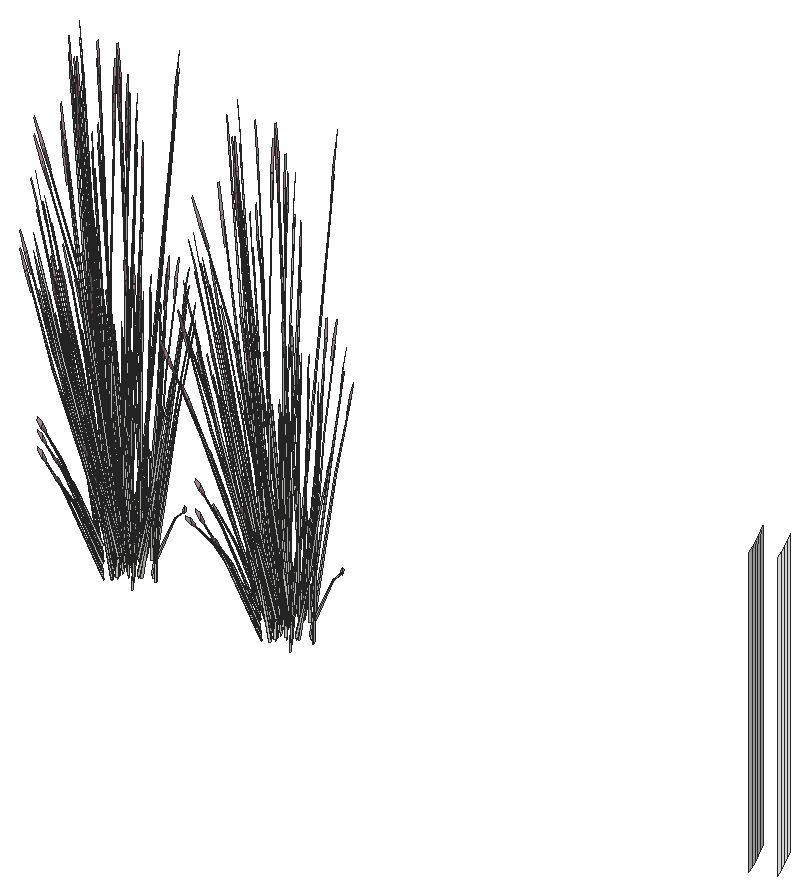
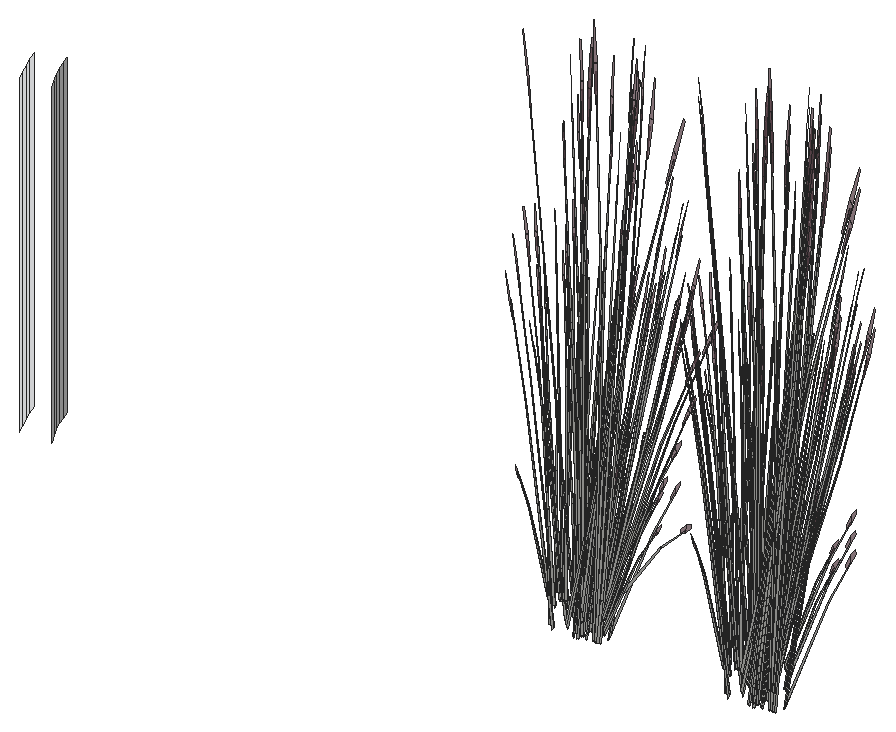
# SketchUp Ruby script. Lengths in inches.
U = 1.inch
M = Sketchup.active_model
def pt(a) = Geom::Point3d.new(a.map { |v| v * U })
def face(e, loops, mat)
  f = e.add_face(loops[0].map { |a| pt(a) })
  loops[1..].each { |l| e.add_face(l.map { |a| pt(a) }).erase! }
  f.material = f.back_material = mat if mat
  f
end
# faces: each face lists its corners as indices into pts; further lists are holes
def faces(e, pts, list, mat = nil) = list.each { |f| face(e, (f[0].is_a?(Array) ? f : [f]).map { |l| l.map { |i| pts[i] } }, mat) }
# xy, xz, yz: faces in a plane at the given z, y or x. An outline is a flat list of corners, or four numbers for a rectangle; further outlines are holes
def ring(l) = l.size == 4 ? [[l[0], l[1]], [l[2], l[1]], [l[2], l[3]], [l[0], l[3]]] : l.each_slice(2).to_a
def flat(e, list, mat, &to3) = list.each { |f| face(e, (f[0].is_a?(Array) ? f : [f]).map { |l| ring(l).map { |u, v| to3.(u, v) } }, mat) }
def xy(e, z, list, mat = nil) = flat(e, list, mat) { |x, y| [x, y, z] }
def xz(e, y, list, mat = nil) = flat(e, list, mat) { |x, z| [x, y, z] }
def yz(e, x, list, mat = nil) = flat(e, list, mat) { |y, z| [x, y, z] }
def lines(e, pts, list) = list.each { |a, b| e.add_line(pt(pts[a]), pt(pts[b])) }
# prism: a flat outline (further loops are holes) pulled along v
def prism(e, loops, v, mat = nil)
  f = face(e, loops, mat); d = Geom::Vector3d.new(v.map { |x| x * U })
  f.pushpull(f.normal.samedirection?(d) ? d.length : -d.length)
end
def box(e, o, s, mat = nil) = prism(e, [[o, [o[0] + s[0], o[1], o[2]], [o[0] + s[0], o[1] + s[1], o[2]], [o[0], o[1] + s[1], o[2]]]], [0, 0, s[2]], mat)
def at(x, y, z, deg = 0) = Geom::Transformation.translation(pt([x, y, z])) * Geom::Transformation.rotation(ORIGIN, Z_AXIS, deg.degrees)
def axes(o, x, y, z) = Geom::Transformation.new([*x, 0, *y, 0, *z, 0, *pt(o).to_a, 1])
def part(name) = M.definitions.add(name)
# library, detail: a bought-in or finely detailed component or shape, given as its bounding box
def library(name, o, s) = part(name).tap { |d| box(d.entities, o, s) }
def detail(e, o, s) = box(e.add_group.entities, o, s)
def put(e, d, t, mat = nil) = e.add_instance(d, t).tap { |i| i.material = mat if mat }
def group(e, t, mat = nil) = e.add_group.tap { |g| g.transformation = t; g.material = mat if mat }.entities
root = M.entities
M.materials.add("Glass_Basic_01").color = [105, 113, 122]
M.materials["Glass_Basic_01"].alpha = 0.25
M.materials.add("LightPink_Translucent").color = [144, 107, 117]
M.materials["LightPink_Translucent"].alpha = 0.75
M.materials.add("M01_Silver_Fog").color = [224, 224, 224]
c1 = part("blade")
p = [[2.15,0.21,22],[0,0.17,0],[0.09,0.45,0],[2.18,0.31,22],[2.29,0.31,22],[0.38,0.45,0],
  [2.48,0.24,33],[2.49,0.24,33],[2.48,0.22,33]]
faces(c1.entities,p,[[0,1,2,3],[4,5,2,3],[6,3,4,7],[8,0,3,6]])
c2 = part("seeds")
p = [[0.3,-0.1,1.38],[-0.01,-0.03,1.59],[-0.01,-0.03,0.03],[0.14,-0.07,-0.07],[0.29,-0.03,3],[0.15,0.01,3.11]]
faces(c2.entities,p,[[0,1,2,3],[1,0,4,5]],"LightPink_Translucent")
c3 = part("blade with seeds")
put(c3.entities,c1,at(0,0,0))
put(c3.entities,c2,axes([2.4,0.25,30.99],[1.5799,-0.05474,1.17369],[-0.12525,1.92788,0.29478],[-0.07173,-0.02425,1.56792]))
p = [[358.13,455.46,648],[358.52,454.41,648],[358.52,454.41,684],[358.13,455.46,684],[361.35,455.41,648],[360.92,456.5625,648],
  [360.92,456.5625,684],[361.35,455.41,684],[357.7,456.49,648],[357.7,456.49,684],[357.23,457.5,648],[357.23,457.5,684],
  [360.45,457.7,648],[360.45,457.7,684],[356.73,458.5,648],[356.73,458.5,684],[359.93,458.82,648],[359.93,458.82,684],
  [356.18,459.47,648],[356.18,459.47,684],[359.37,459.91,648],[359.37,459.91,684]]
faces(root,p,[[0,1,2,3],[8,0,3,9],[10,8,9,11],[14,10,11,15],[18,14,15,19]],"M01_Silver_Fog")
faces(root,p,[[4,5,6,7],[5,12,13,6],[12,16,17,13],[16,20,21,17]],"Glass_Basic_01")
put(root,c3,axes([273.62,459.22,653.09],[0.41494,-0.39744,0.53763],[0.35786,0.42207,0.4433],[-0.19468,-0.07331,1.11249]))
put(root,c3,axes([273.81,459.22,652.73],[0.0253,-0.40952,0.0643],[0.38204,0.01123,0.50621],[-0.14634,-0.04285,0.77189]))
put(root,c3,axes([274.98,458.51,653.43],[-0.33533,0.51628,-0.13619],[-0.48563,-0.29744,-0.75594],[-0.16881,-0.14586,1.14864]))
put(root,c3,axes([274.07,459.53,653.05],[0.28589,0.33718,0.35414],[-0.32644,0.31919,-0.4572],[-0.16586,-0.04856,0.87481]))
put(root,c3,axes([274.84,458.93,652.98],[-0.42844,-0.2603,-0.71045],[0.30448,-0.45614,0.08574],[-0.15523,-0.15542,1.00501]))
put(root,c3,axes([274.84,458.93,654.98],[-0.42844,-0.2603,-0.71045],[0.30448,-0.45614,0.08574],[-0.15523,-0.15542,1.00501]))
put(root,c3,axes([274.64,458.94,652.68],[-0.4958,0.12802,-0.51099],[-0.08673,-0.48481,-0.3958],[-0.13317,-0.13893,0.97773]))
put(root,c3,axes([274.64,458.94,654.68],[-0.4958,0.12802,-0.51099],[-0.08673,-0.48481,-0.3958],[-0.13317,-0.13893,0.97773]))
put(root,c3,axes([274,458.5,649.49],[-0.04867,0.07094,1.76342],[-0.49185,0.15296,-0.26939],[-0.11882,-0.13915,0.30037]))
put(root,c3,axes([274,458.5,651.49],[-0.04867,0.07094,1.76342],[-0.49185,0.15296,-0.26939],[-0.11882,-0.13915,0.30037]))
put(root,c3,axes([273.69,458.77,650.13],[-0.14494,0.43975,-0.03893],[-0.4461,-0.13527,-0.17649],[-0.06773,-0.07192,0.58215]))
put(root,c3,axes([273.69,458.77,652.13],[-0.14494,0.43975,-0.03893],[-0.4461,-0.13527,-0.17649],[-0.06773,-0.07192,0.58215]))
put(root,c3,axes([274.86,457.28,652.71],[-0.00937,0.06455,1.77383],[-0.46231,0.23427,-0.16761],[-0.13604,-0.11975,0.31391]))
put(root,c3,axes([274.69,458.59,652.53],[-0.0776,-0.43378,-0.35414],[0.44361,-0.11454,0.4572],[-0.11915,-0.12431,0.87481]))
put(root,c3,axes([274.69,458.59,654.53],[-0.0776,-0.43378,-0.35414],[0.44361,-0.11454,0.4572],[-0.11915,-0.12431,0.87481]))
put(root,c3,axes([273.45,460.78,650.375],[-0.62828,0,0],[0,-0.6019,-0.51607],[0,-0.13709,1.63711]))
put(root,c3,axes([273.45,460.78,652.375],[-0.62828,0,0],[0,-0.6019,-0.51607],[0,-0.13709,1.63711]))
put(root,c3,axes([274.95,458.94,653.05],[0.0776,0.43378,0.35414],[-0.44361,0.11454,-0.4572],[-0.11915,-0.12431,0.87481]))
put(root,c3,axes([273.94,460.625,650.33],[-0.46736,0.45277,0.30756],[-0.46764,-0.44801,-0.36492],[-0.01632,-0.12858,1.64885]))
put(root,c3,axes([273.94,460.625,652.33],[-0.46736,0.45277,0.30756],[-0.46764,-0.44801,-0.36492],[-0.01632,-0.12858,1.64885]))
put(root,c3,axes([275.86,461.875,651.33],[0.4342,0.21716,1.51261],[-0.42537,0.46784,0.59816],[-0.19053,-0.27728,1.26806]))
put(root,c3,axes([275.86,461.875,653.33],[0.4342,0.21716,1.51261],[-0.42537,0.46784,0.59816],[-0.19053,-0.27728,1.26806]))
put(root,c3,axes([274.21,457.9375,650.77],[0.2621,0.18744,1.1486],[-0.38171,0.11267,0.84392],[-0.08167,-0.14405,0.25299]))
put(root,c3,axes([274.21,457.9375,652.77],[0.2621,0.18744,1.1486],[-0.38171,0.11267,0.84392],[-0.08167,-0.14405,0.25299]))
put(root,c3,axes([275.16,461.31,650.21],[-0.30184,-0.45202,-0.44739],[0.45719,-0.31831,0.21531],[-0.09768,-0.05593,1.43643]))
put(root,c3,axes([275.16,461.31,652.21],[-0.30184,-0.45202,-0.44739],[0.45719,-0.31831,0.21531],[-0.09768,-0.05593,1.43643]))
put(root,c3,axes([274.75,458.43,653.09],[0.55971,-0.13842,0.53763],[0.09714,0.54299,0.4433],[-0.13164,-0.16003,1.11249]))
put(root,c3,axes([274.88,458.55,652.73],[0.22836,-0.34211,0.0643],[0.3252,0.19918,0.50621],[-0.10513,-0.10968,0.77189]))
put(root,c3,axes([275.21,461.57,650.4375],[0.13317,-0.63814,-0.23429],[0.63143,0.11124,0.51271],[-0.11033,-0.08813,1.5644]))
put(root,c3,axes([275.21,461.57,652.4375],[0.13317,-0.63814,-0.23429],[0.63143,0.11124,0.51271],[-0.11033,-0.08813,1.5644]))
put(root,c3,axes([273.59,460.375,650.02],[0,-0.53854,-0.49651],[0.56215,0,0],[0,-0.12266,1.57504]))
put(root,c3,axes([273.59,460.375,652.02],[0,-0.53854,-0.49651],[0.56215,0,0],[0,-0.12266,1.57504]))
put(root,c3,axes([273.83,460.875,650.48],[0,0.53854,0.49651],[-0.56215,0,0],[0,-0.12266,1.57504]))
put(root,c3,axes([273.83,460.875,652.48],[0,0.53854,0.49651],[-0.56215,0,0],[0,-0.12266,1.57504]))
put(root,c3,axes([275.0625,461,650.67],[-0.56585,-0.25696,-0.29095],[0.27246,-0.54236,-0.50002],[-0.01778,-0.13316,1.59708]))
put(root,c3,axes([275.0625,461,652.67],[-0.56585,-0.25696,-0.29095],[0.27246,-0.54236,-0.50002],[-0.01778,-0.13316,1.59708]))
put(root,c3,axes([274.81,460.45,650.1],[-0.20635,-0.55225,-0.69835],[0.59439,-0.19889,-0.18329],[-0.02281,-0.18701,1.54149]))
put(root,c3,axes([274.81,460.45,652.1],[-0.20635,-0.55225,-0.69835],[0.59439,-0.19889,-0.18329],[-0.02281,-0.18701,1.54149]))
put(root,c3,axes([276.16,458.7,653.03],[-0.49168,0.25073,-0.1216],[-0.24162,-0.44501,-0.67495],[-0.06487,-0.18753,1.02557]))
put(root,c3,axes([275.74,458.72,652.68],[-0.49392,-0.135,-0.51099],[0.1693,-0.46287,-0.3958],[-0.04529,-0.18636,0.97773]))
put(root,c3,axes([275.74,458.72,654.68],[-0.49392,-0.135,-0.51099],[0.1693,-0.46287,-0.3958],[-0.04529,-0.18636,0.97773]))
put(root,c3,axes([273.83,460.39,650.03],[0.35073,-0.33601,-0.30978],[0.35073,0.33601,0.30978],[0,-0.10823,1.38974]))
put(root,c3,axes([273.83,460.39,652.03],[0.35073,-0.33601,-0.30978],[0.35073,0.33601,0.30978],[0,-0.10823,1.38974]))
put(root,c3,axes([275.42,458.21,650.13],[-0.34721,0.30895,-0.03893],[-0.31814,-0.33837,-0.17649],[-0.0224,-0.09588,0.58215]))
put(root,c3,axes([275.42,458.21,652.13],[-0.34721,0.30895,-0.03893],[-0.31814,-0.33837,-0.17649],[-0.0224,-0.09588,0.58215]))
put(root,c3,axes([276.01,458.87,653.05],[-0.15148,0.41415,0.35414],[-0.44193,-0.12079,-0.4572],[-0.04052,-0.16674,0.87481]))
put(root,c3,axes([275.96,458.43,652.53],[0.15148,-0.41415,-0.35414],[0.44193,0.12079,0.4572],[-0.04052,-0.16674,0.87481]))
put(root,c3,axes([275.96,458.43,654.53],[0.15148,-0.41415,-0.35414],[0.44193,0.12079,0.4572],[-0.04052,-0.16674,0.87481]))
put(root,c3,axes([275.22,460.67,650.36],[0.21845,0.6022,0.45755],[-0.62418,0.20941,0.17955],[0.00763,-0.11065,1.58856]))
put(root,c3,axes([275.22,460.67,652.36],[0.21845,0.6022,0.45755],[-0.62418,0.20941,0.17955],[0.00763,-0.11065,1.58856]))
put(root,c3,axes([275.125,460.59,650.21],[0.24378,-0.48527,-0.44739],[0.50654,0.23354,0.21531],[0,-0.11186,1.43643]))
put(root,c3,axes([275.125,460.59,652.21],[0.24378,-0.48527,-0.44739],[0.50654,0.23354,0.21531],[0,-0.11186,1.43643]))
put(root,c3,axes([276.15,458.5,652.73],[0.37023,-0.18303,0.0643],[0.18122,0.33376,0.50621],[-0.03575,-0.14712,0.77189]))
put(root,c3,axes([276.02,458.53,652.73],[0.4951,0.14079,0.48003],[-0.1693,0.46287,0.3958],[-0.02975,-0.18203,0.9933]))
put(root,c3,axes([275.43,460.83,650.43],[0.56613,0.26102,0.24065],[-0.27246,0.54236,0.50002],[0,-0.12502,1.60543]))
put(root,c3,axes([275.43,460.83,652.43],[0.56613,0.26102,0.24065],[-0.27246,0.54236,0.50002],[0,-0.12502,1.60543]))
put(root,c3,axes([275.24,460.47,650.72],[-0.54562,0.03324,0.44739],[-0.04934,-0.55185,-0.21531],[0.09768,-0.05593,1.43643]))
put(root,c3,axes([275.24,460.47,652.72],[-0.54562,0.03324,0.44739],[-0.04934,-0.55185,-0.21531],[0.09768,-0.05593,1.43643]))
put(root,c3,axes([274.73,458.86,650.375],[-0.31414,-0.53965,0],[0.52557,-0.30095,-0.51607],[0.1197,-0.06854,1.63711]))
put(root,c3,axes([274.73,458.86,652.375],[-0.31414,-0.53965,0],[0.52557,-0.30095,-0.51607],[0.1197,-0.06854,1.63711]))
put(root,c3,axes([276.04,457.56,650.77],[0.06446,0.31404,1.1486],[-0.35756,-0.17393,0.84392],[0.03848,-0.1608,0.25299]))
put(root,c3,axes([276.04,457.56,652.77],[0.06446,0.31404,1.1486],[-0.35756,-0.17393,0.84392],[0.03848,-0.1608,0.25299]))
put(root,c3,axes([277.58,458.07,652.71],[-0.05103,0.04113,1.77383],[-0.49994,-0.13878,-0.16761],[-0.0181,-0.17951,0.31391]))
put(root,c3,axes([277.18,459.26,653.03],[-0.55221,-0.02668,-0.1216],[0.01509,-0.50521,-0.67495],[0.03836,-0.19458,1.02557]))
put(root,c3,axes([276.97,459.34,653.05],[-0.33997,0.28354,0.35414],[-0.32182,-0.32376,-0.4572],[0.04897,-0.1645,0.87481]))
put(root,c3,axes([275.35,460.35,650.67],[-0.05855,-0.61451,-0.29095],[0.60981,-0.03716,-0.50002],[0.10738,-0.08185,1.59708]))
put(root,c3,axes([275.35,460.35,652.67],[-0.05855,-0.61451,-0.29095],[0.60981,-0.03716,-0.50002],[0.10738,-0.08185,1.59708]))
put(root,c3,axes([276.81,459.07,652.68],[-0.35968,-0.36185,-0.51099],[0.37996,-0.3169,-0.3958],[0.05473,-0.18385,0.97773]))
put(root,c3,axes([276.81,459.07,654.68],[-0.35968,-0.36185,-0.51099],[0.37996,-0.3169,-0.3958],[0.05473,-0.18385,0.97773]))
put(root,c3,axes([275.27,458.99,650.03],[0.46876,0.13325,-0.30978],[-0.11803,0.46926,0.30978],[0.0945,-0.05411,1.38974]))
put(root,c3,axes([275.27,458.99,652.03],[0.46876,0.13325,-0.30978],[-0.11803,0.46926,0.30978],[0.0945,-0.05411,1.38974]))
put(root,c3,axes([275.16,458.78,650.02],[0.47024,-0.26927,-0.49651],[0.28107,0.48284,0],[0.1071,-0.06133,1.57504]))
put(root,c3,axes([275.16,458.78,652.02],[0.47024,-0.26927,-0.49651],[0.28107,0.48284,0],[0.1071,-0.06133,1.57504]))
put(root,c3,axes([277.14,458.93,652.53],[0.33997,-0.28354,-0.35414],[0.32182,0.32376,0.4572],[0.04897,-0.1645,0.87481]))
put(root,c3,axes([277.14,458.93,654.53],[0.33997,-0.28354,-0.35414],[0.32182,0.32376,0.4572],[0.04897,-0.1645,0.87481]))
put(root,c3,axes([277.27,459.08,652.73],[0.4129,0.02509,0.0643],[-0.01132,0.37891,0.50621],[0.04321,-0.14514,0.77189]))
put(root,c3,axes([275.71,459.88,650.06],[0.33843,-0.40479,-0.62353],[0.42041,0.36705,-0.16365],[0.13561,-0.10098,1.37633]))
put(root,c3,axes([275.71,459.88,652.06],[0.33843,-0.40479,-0.62353],[0.42041,0.36705,-0.16365],[0.13561,-0.10098,1.37633]))
put(root,c3,axes([277.14,459.05,652.73],[0.35779,0.36745,0.48003],[-0.37996,0.3169,0.3958],[0.066,-0.17239,0.9933]))
put(root,c3,axes([277.56,460.21,653.05],[-0.43736,0.07697,0.35414],[-0.11549,-0.43998,-0.4572],[0.12533,-0.11818,0.87481]))
put(root,c3,axes([276.3,458.98,651.875],[-0.09355,0.18511,1.71376],[-0.39247,-0.38307,0.13857],[0.17705,-0.23875,0.73262]))
put(root,c3,axes([276.3,458.98,653.875],[-0.09355,0.18511,1.71376],[-0.39247,-0.38307,0.13857],[0.17705,-0.23875,0.73262]))
put(root,c3,axes([277.78,460.25,653.03],[-0.46478,-0.29695,-0.1216],[0.26776,-0.43004,-0.67495],[0.13131,-0.14949,1.02557]))
put(root,c3,axes([277.04,459,650.375],[0.31414,-0.53965,0],[0.52557,0.30095,-0.51607],[0.1197,0.06854,1.63711]))
put(root,c3,axes([277.04,459,652.375],[0.31414,-0.53965,0],[0.52557,0.30095,-0.51607],[0.1197,0.06854,1.63711]))
put(root,c3,axes([277.57,458.76,649.49],[-0.0752,-0.04243,1.76342],[-0.19317,-0.47398,-0.26939],[0.13031,-0.12863,0.30037]))
put(root,c3,axes([277.57,458.76,651.49],[-0.0752,-0.04243,1.76342],[-0.19317,-0.47398,-0.26939],[0.13031,-0.12863,0.30037]))
put(root,c3,axes([277.55,459.9,652.68],[-0.12908,-0.49174,-0.51099],[0.48882,-0.08602,-0.3958],[0.14008,-0.13208,0.97773]))
put(root,c3,axes([277.55,459.9,654.68],[-0.12908,-0.49174,-0.51099],[0.48882,-0.08602,-0.3958],[0.14008,-0.13208,0.97773]))
put(root,c3,axes([278.87,460.68,650.26],[-0.31151,-0.34437,-0.06488],[0.34117,-0.31553,-0.29416],[0.09667,-0.02221,0.97024]))
put(root,c3,axes([278.87,460.68,652.26],[-0.31151,-0.34437,-0.06488],[0.34117,-0.31553,-0.29416],[0.09667,-0.02221,0.97024]))
put(root,c3,axes([278.15,458.92,650.77],[-0.16736,0.27414,1.1486],[-0.14385,-0.36832,0.84392],[0.13822,-0.09229,0.25299]))
put(root,c3,axes([278.15,458.92,652.77],[-0.16736,0.27414,1.1486],[-0.14385,-0.36832,0.84392],[0.13822,-0.09229,0.25299]))
put(root,c3,axes([277.95,460.14,652.73],[0.34493,0.22649,0.0643],[-0.20082,0.32253,0.50621],[0.11059,-0.10427,0.77189]))
put(root,c3,axes([277.86,460.05,652.73],[0.12461,0.49565,0.48003],[-0.48882,0.08602,0.3958],[0.14406,-0.11657,0.9933]))
put(root,c3,axes([278.93,460.125,652.71],[-0.06563,-0.00409,1.77383],[-0.27252,-0.43825,-0.16761],[0.10944,-0.1441,0.31391]))
put(root,c3,axes([277.91,459.95,652.53],[0.43736,-0.07697,-0.35414],[0.11549,0.43998,0.4572],[0.12533,-0.11818,0.87481]))
put(root,c3,axes([277.91,459.95,654.53],[0.43736,-0.07697,-0.35414],[0.11549,0.43998,0.4572],[0.12533,-0.11818,0.87481]))
put(root,c3,axes([277.57,460.1,652.98],[0.26246,-0.42493,-0.71045],[0.45991,0.30199,0.08574],[0.15671,-0.15395,1.00501]))
put(root,c3,axes([277.57,460.1,654.98],[0.26246,-0.42493,-0.71045],[0.45991,0.30199,0.08574],[0.15671,-0.15395,1.00501]))
put(root,c3,axes([277.8,461.41,653.03],[-0.25281,-0.48765,-0.1216],[0.44869,-0.23964,-0.67495],[0.18908,-0.06434,1.02557]))
put(root,c3,axes([277.78,460.99,652.68],[0.13612,-0.48987,-0.51099],[0.46669,0.16791,-0.3958],[0.1879,-0.04492,0.97773]))
put(root,c3,axes([277.78,460.99,654.68],[0.13612,-0.48987,-0.51099],[0.46669,0.16791,-0.3958],[0.1879,-0.04492,0.97773]))
put(root,c3,axes([277.95,459.71,650.59],[-0.1795,-0.01595,1.43002],[-0.18389,-0.42791,-0.30754],[0.22051,-0.12105,0.61141]))
put(root,c3,axes([277.95,459.71,652.59],[-0.1795,-0.01595,1.43002],[-0.18389,-0.42791,-0.30754],[0.22051,-0.12105,0.61141]))
put(root,c3,axes([278.28,461.13,649.98],[-0.32361,0.06463,1.41583],[-0.05151,-0.51444,0.08104],[0.22666,-0.07786,0.80566]))
put(root,c3,axes([278.28,461.13,651.98],[-0.32361,0.06463,1.41583],[-0.05151,-0.51444,0.08104],[0.22666,-0.07786,0.80566]))
put(root,c3,axes([279.18,460.65,652.72],[0.06972,-0.08203,1.74944],[-0.08924,-0.50318,-0.27667],[0.17494,-0.0954,0.14031]))
put(root,c3,axes([293.24,460.07,651.875],[0.20841,-0.0122,1.71376],[-0.13825,0.52864,0.13857],[-0.297,-0.0327,0.73262]))
put(root,c3,axes([293.86,459.57,652.98],[-0.50227,-0.01297,-0.71045],[0.03373,-0.54602,0.08574],[-0.21278,-0.05762,1.00501]))
put(root,c3,axes([293.46,459.71,650.59],[0.0981,0.14994,1.43002],[-0.22605,0.40756,-0.30754],[-0.23211,-0.09741,0.61141]))
put(root,c3,axes([293.63,459.22,651.875],[0.18664,0.09279,1.71376],[-0.38624,0.38925,0.13857],[-0.24072,-0.1756,0.73262]))
put(root,c3,axes([293.69,459.68,652.68],[-0.36484,0.35674,-0.51099],[-0.31952,-0.37685,-0.3958],[-0.18537,-0.05428,0.97773]))
put(root,c3,axes([293.18,458.68,652.71],[0.03725,0.05374,1.77383],[-0.17957,0.48312,-0.16761],[-0.18186,0.0035,0.31391]))
put(root,c3,axes([293.59,458.36,652.72],[-0.10811,-0.0038,1.74944],[-0.34418,0.38014,-0.27667],[-0.18364,-0.07767,0.14031]))
put(root,c3,axes([293.89,459.3125,653.03],[-0.0269,0.54769,-0.1216],[-0.50939,-0.01497,-0.67495],[-0.19618,-0.03804,1.02557]))
put(root,c3,axes([293.56,459.35,652.53],[-0.28589,-0.33718,-0.35414],[0.32644,-0.31919,0.4572],[-0.16586,-0.04856,0.87481]))
put(root,c3,axes([292.87,460.16,650.77],[0.32078,-0.03854,1.1486],[-0.20348,0.33954,0.84392],[-0.15852,-0.05093,0.25299]))
put(root,c3,axes([293.52,459.22,653.09],[0.41494,-0.39744,0.53763],[0.35786,0.42207,0.4433],[-0.19468,-0.07331,1.11249]))
put(root,c3,axes([293.7,459.22,652.73],[0.0253,-0.40952,0.0643],[0.38204,0.01123,0.50621],[-0.14634,-0.04285,0.77189]))
put(root,c3,axes([294.88,458.51,653.43],[-0.33533,0.51628,-0.13619],[-0.48563,-0.29744,-0.75594],[-0.16881,-0.14586,1.14864]))
put(root,c3,axes([293.96,459.53,653.05],[0.28589,0.33718,0.35414],[-0.32644,0.31919,-0.4572],[-0.16586,-0.04856,0.87481]))
put(root,c3,axes([294.73,458.93,652.98],[-0.42844,-0.2603,-0.71045],[0.30448,-0.45614,0.08574],[-0.15523,-0.15542,1.00501]))
put(root,c3,axes([294.53,458.94,652.68],[-0.4958,0.12802,-0.51099],[-0.08673,-0.48481,-0.3958],[-0.13317,-0.13893,0.97773]))
put(root,c3,axes([293.89,458.5,649.49],[-0.04867,0.07094,1.76342],[-0.49185,0.15296,-0.26939],[-0.11882,-0.13915,0.30037]))
put(root,c3,axes([293.59,458.77,650.13],[-0.14494,0.43975,-0.03893],[-0.4461,-0.13527,-0.17649],[-0.06773,-0.07192,0.58215]))
put(root,c3,axes([294.75,457.28,652.71],[-0.00937,0.06455,1.77383],[-0.46231,0.23427,-0.16761],[-0.13604,-0.11975,0.31391]))
put(root,c3,axes([294.59,458.59,652.53],[-0.0776,-0.43378,-0.35414],[0.44361,-0.11454,0.4572],[-0.11915,-0.12431,0.87481]))
put(root,c3,axes([293.35,460.78,650.375],[-0.62828,0,0],[0,-0.6019,-0.51607],[0,-0.13709,1.63711]))
put(root,c3,axes([294.85,458.94,653.05],[0.0776,0.43378,0.35414],[-0.44361,0.11454,-0.4572],[-0.11915,-0.12431,0.87481]))
put(root,c3,axes([293.83,460.625,650.33],[-0.46736,0.45277,0.30756],[-0.46764,-0.44801,-0.36492],[-0.01632,-0.12858,1.64885]))
put(root,c3,axes([295.76,461.875,651.33],[0.4342,0.21716,1.51261],[-0.42537,0.46784,0.59816],[-0.19053,-0.27728,1.26806]))
put(root,c3,axes([294.1,457.9375,650.77],[0.2621,0.18744,1.1486],[-0.38171,0.11267,0.84392],[-0.08167,-0.14405,0.25299]))
put(root,c3,axes([295.06,461.31,650.21],[-0.30184,-0.45202,-0.44739],[0.45719,-0.31831,0.21531],[-0.09768,-0.05593,1.43643]))
put(root,c3,axes([294.65,458.43,653.09],[0.55971,-0.13842,0.53763],[0.09714,0.54299,0.4433],[-0.13164,-0.16003,1.11249]))
put(root,c3,axes([294.78,458.55,652.73],[0.22836,-0.34211,0.0643],[0.3252,0.19918,0.50621],[-0.10513,-0.10968,0.77189]))
put(root,c3,axes([295.1,461.57,650.4375],[0.13317,-0.63814,-0.23429],[0.63143,0.11124,0.51271],[-0.11033,-0.08813,1.5644]))
put(root,c3,axes([293.49,460.375,650.02],[0,-0.53854,-0.49651],[0.56215,0,0],[0,-0.12266,1.57504]))
put(root,c3,axes([293.73,460.875,650.48],[0,0.53854,0.49651],[-0.56215,0,0],[0,-0.12266,1.57504]))
put(root,c3,axes([294.96,461,650.67],[-0.56585,-0.25696,-0.29095],[0.27246,-0.54236,-0.50002],[-0.01778,-0.13316,1.59708]))
put(root,c3,axes([294.71,460.45,650.1],[-0.20635,-0.55225,-0.69835],[0.59439,-0.19889,-0.18329],[-0.02281,-0.18701,1.54149]))
put(root,c3,axes([296.06,458.7,653.03],[-0.49168,0.25073,-0.1216],[-0.24162,-0.44501,-0.67495],[-0.06487,-0.18753,1.02557]))
put(root,c3,axes([295.63,458.72,652.68],[-0.49392,-0.135,-0.51099],[0.1693,-0.46287,-0.3958],[-0.04529,-0.18636,0.97773]))
put(root,c3,axes([293.73,460.39,650.03],[0.35073,-0.33601,-0.30978],[0.35073,0.33601,0.30978],[0,-0.10823,1.38974]))
put(root,c3,axes([295.3125,458.21,650.13],[-0.34721,0.30895,-0.03893],[-0.31814,-0.33837,-0.17649],[-0.0224,-0.09588,0.58215]))
put(root,c3,axes([295.91,458.87,653.05],[-0.15148,0.41415,0.35414],[-0.44193,-0.12079,-0.4572],[-0.04052,-0.16674,0.87481]))
put(root,c3,axes([295.86,458.43,652.53],[0.15148,-0.41415,-0.35414],[0.44193,0.12079,0.4572],[-0.04052,-0.16674,0.87481]))
put(root,c3,axes([295.12,460.67,650.36],[0.21845,0.6022,0.45755],[-0.62418,0.20941,0.17955],[0.00763,-0.11065,1.58856]))
put(root,c3,axes([295.02,460.59,650.21],[0.24378,-0.48527,-0.44739],[0.50654,0.23354,0.21531],[0,-0.11186,1.43643]))
put(root,c3,axes([296.05,458.5,652.73],[0.37023,-0.18303,0.0643],[0.18122,0.33376,0.50621],[-0.03575,-0.14712,0.77189]))
put(root,c3,axes([295.91,458.53,652.73],[0.4951,0.14079,0.48003],[-0.1693,0.46287,0.3958],[-0.02975,-0.18203,0.9933]))
put(root,c3,axes([295.32,460.83,650.43],[0.56613,0.26102,0.24065],[-0.27246,0.54236,0.50002],[0,-0.12502,1.60543]))
put(root,c3,axes([295.14,460.47,650.72],[-0.54562,0.03324,0.44739],[-0.04934,-0.55185,-0.21531],[0.09768,-0.05593,1.43643]))
put(root,c3,axes([294.625,458.86,650.375],[-0.31414,-0.53965,0],[0.52557,-0.30095,-0.51607],[0.1197,-0.06854,1.63711]))
put(root,c3,axes([295.9375,457.56,650.77],[0.06446,0.31404,1.1486],[-0.35756,-0.17393,0.84392],[0.03848,-0.1608,0.25299]))
put(root,c3,axes([297.47,458.07,652.71],[-0.05103,0.04113,1.77383],[-0.49994,-0.13878,-0.16761],[-0.0181,-0.17951,0.31391]))
put(root,c3,axes([297.08,459.26,653.03],[-0.55221,-0.02668,-0.1216],[0.01509,-0.50521,-0.67495],[0.03836,-0.19458,1.02557]))
put(root,c3,axes([296.86,459.34,653.05],[-0.33997,0.28354,0.35414],[-0.32182,-0.32376,-0.4572],[0.04897,-0.1645,0.87481]))
put(root,c3,axes([295.24,460.35,650.67],[-0.05855,-0.61451,-0.29095],[0.60981,-0.03716,-0.50002],[0.10738,-0.08185,1.59708]))
put(root,c3,axes([296.7,459.07,652.68],[-0.35968,-0.36185,-0.51099],[0.37996,-0.3169,-0.3958],[0.05473,-0.18385,0.97773]))
put(root,c3,axes([295.16,458.99,650.03],[0.46876,0.13325,-0.30978],[-0.11803,0.46926,0.30978],[0.0945,-0.05411,1.38974]))
put(root,c3,axes([295.05,458.78,650.02],[0.47024,-0.26927,-0.49651],[0.28107,0.48284,0],[0.1071,-0.06133,1.57504]))
put(root,c3,axes([297.04,458.93,652.53],[0.33997,-0.28354,-0.35414],[0.32182,0.32376,0.4572],[0.04897,-0.1645,0.87481]))
put(root,c3,axes([297.17,459.08,652.73],[0.4129,0.02509,0.0643],[-0.01132,0.37891,0.50621],[0.04321,-0.14514,0.77189]))
put(root,c3,axes([295.61,459.88,650.06],[0.33843,-0.40479,-0.62353],[0.42041,0.36705,-0.16365],[0.13561,-0.10098,1.37633]))
put(root,c3,axes([297.04,459.05,652.73],[0.35779,0.36745,0.48003],[-0.37996,0.3169,0.3958],[0.066,-0.17239,0.9933]))
put(root,c3,axes([297.45,460.21,653.05],[-0.43736,0.07697,0.35414],[-0.11549,-0.43998,-0.4572],[0.12533,-0.11818,0.87481]))
put(root,c3,axes([296.19,458.98,651.875],[-0.09355,0.18511,1.71376],[-0.39247,-0.38307,0.13857],[0.17705,-0.23875,0.73262]))
put(root,c3,axes([297.68,460.25,653.03],[-0.46478,-0.29695,-0.1216],[0.26776,-0.43004,-0.67495],[0.13131,-0.14949,1.02557]))
put(root,c3,axes([296.9375,459,650.375],[0.31414,-0.53965,0],[0.52557,0.30095,-0.51607],[0.1197,0.06854,1.63711]))
put(root,c3,axes([297.46,458.76,649.49],[-0.0752,-0.04243,1.76342],[-0.19317,-0.47398,-0.26939],[0.13031,-0.12863,0.30037]))
put(root,c3,axes([297.45,459.9,652.68],[-0.12908,-0.49174,-0.51099],[0.48882,-0.08602,-0.3958],[0.14008,-0.13208,0.97773]))
put(root,c3,axes([298.76,460.68,650.26],[-0.31151,-0.34437,-0.06488],[0.34117,-0.31553,-0.29416],[0.09667,-0.02221,0.97024]))
put(root,c3,axes([298.05,458.92,650.77],[-0.16736,0.27414,1.1486],[-0.14385,-0.36832,0.84392],[0.13822,-0.09229,0.25299]))
put(root,c3,axes([297.85,460.14,652.73],[0.34493,0.22649,0.0643],[-0.20082,0.32253,0.50621],[0.11059,-0.10427,0.77189]))
put(root,c3,axes([297.75,460.05,652.73],[0.12461,0.49565,0.48003],[-0.48882,0.08602,0.3958],[0.14406,-0.11657,0.9933]))
put(root,c3,axes([298.82,460.125,652.71],[-0.06563,-0.00409,1.77383],[-0.27252,-0.43825,-0.16761],[0.10944,-0.1441,0.31391]))
put(root,c3,axes([297.81,459.95,652.53],[0.43736,-0.07697,-0.35414],[0.11549,0.43998,0.4572],[0.12533,-0.11818,0.87481]))
put(root,c3,axes([297.46,460.1,652.98],[0.26246,-0.42493,-0.71045],[0.45991,0.30199,0.08574],[0.15671,-0.15395,1.00501]))
put(root,c3,axes([297.7,461.41,653.03],[-0.25281,-0.48765,-0.1216],[0.44869,-0.23964,-0.67495],[0.18908,-0.06434,1.02557]))
put(root,c3,axes([297.68,460.99,652.68],[0.13612,-0.48987,-0.51099],[0.46669,0.16791,-0.3958],[0.1879,-0.04492,0.97773]))
put(root,c3,axes([297.84,459.71,650.59],[-0.1795,-0.01595,1.43002],[-0.18389,-0.42791,-0.30754],[0.22051,-0.12105,0.61141]))
put(root,c3,axes([298.17,461.13,649.98],[-0.32361,0.06463,1.41583],[-0.05151,-0.51444,0.08104],[0.22666,-0.07786,0.80566]))
put(root,c3,axes([299.07,460.65,652.72],[0.06972,-0.08203,1.74944],[-0.08924,-0.50318,-0.27667],[0.17494,-0.0954,0.14031]))
